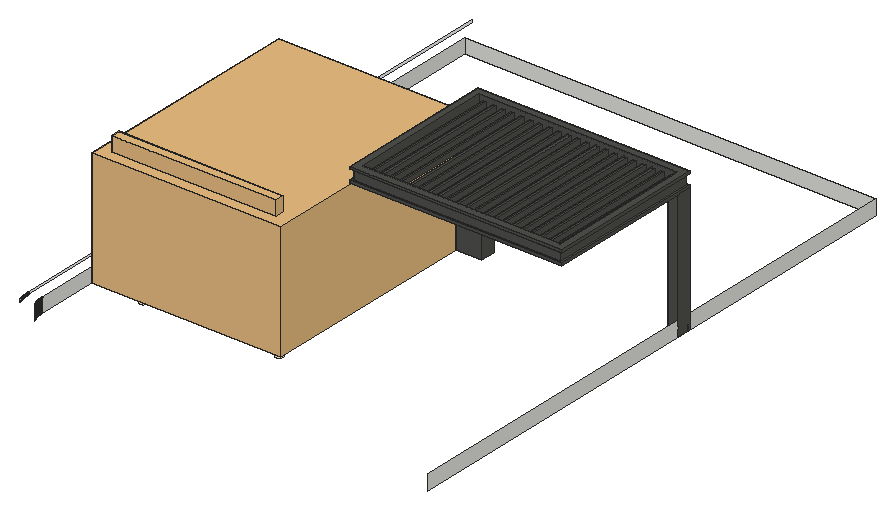
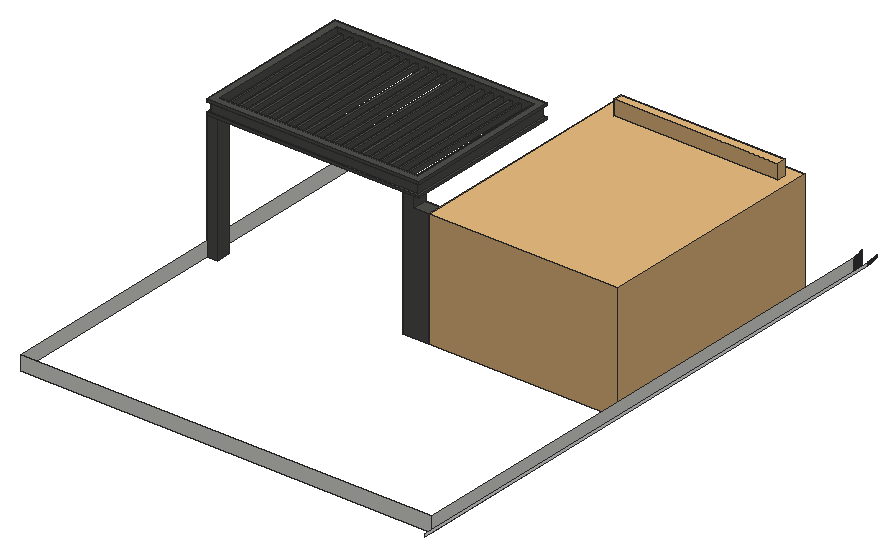
# SketchUp Ruby script. Lengths in inches.
U = 1.inch
M = Sketchup.active_model
def pt(a) = Geom::Point3d.new(a.map { |v| v * U })
def face(e, loops, mat)
  f = e.add_face(loops[0].map { |a| pt(a) })
  loops[1..].each { |l| e.add_face(l.map { |a| pt(a) }).erase! }
  f.material = f.back_material = mat if mat
  f
end
# faces: each face lists its corners as indices into pts; further lists are holes
def faces(e, pts, list, mat = nil) = list.each { |f| face(e, (f[0].is_a?(Array) ? f : [f]).map { |l| l.map { |i| pts[i] } }, mat) }
# xy, xz, yz: faces in a plane at the given z, y or x. An outline is a flat list of corners, or four numbers for a rectangle; further outlines are holes
def ring(l) = l.size == 4 ? [[l[0], l[1]], [l[2], l[1]], [l[2], l[3]], [l[0], l[3]]] : l.each_slice(2).to_a
def flat(e, list, mat, &to3) = list.each { |f| face(e, (f[0].is_a?(Array) ? f : [f]).map { |l| ring(l).map { |u, v| to3.(u, v) } }, mat) }
def xy(e, z, list, mat = nil) = flat(e, list, mat) { |x, y| [x, y, z] }
def xz(e, y, list, mat = nil) = flat(e, list, mat) { |x, z| [x, y, z] }
def yz(e, x, list, mat = nil) = flat(e, list, mat) { |y, z| [x, y, z] }
def lines(e, pts, list) = list.each { |a, b| e.add_line(pt(pts[a]), pt(pts[b])) }
# prism: a flat outline (further loops are holes) pulled along v
def prism(e, loops, v, mat = nil)
  f = face(e, loops, mat); d = Geom::Vector3d.new(v.map { |x| x * U })
  f.pushpull(f.normal.samedirection?(d) ? d.length : -d.length)
end
def box(e, o, s, mat = nil) = prism(e, [[o, [o[0] + s[0], o[1], o[2]], [o[0] + s[0], o[1] + s[1], o[2]], [o[0], o[1] + s[1], o[2]]]], [0, 0, s[2]], mat)
def at(x, y, z, deg = 0) = Geom::Transformation.translation(pt([x, y, z])) * Geom::Transformation.rotation(ORIGIN, Z_AXIS, deg.degrees)
def axes(o, x, y, z) = Geom::Transformation.new([*x, 0, *y, 0, *z, 0, *pt(o).to_a, 1])
def part(name) = M.definitions.add(name)
# library, detail: a bought-in or finely detailed component or shape, given as its bounding box
def library(name, o, s) = part(name).tap { |d| box(d.entities, o, s) }
def detail(e, o, s) = box(e.add_group.entities, o, s)
def put(e, d, t, mat = nil) = e.add_instance(d, t).tap { |i| i.material = mat if mat }
def group(e, t, mat = nil) = e.add_group.tap { |g| g.transformation = t; g.material = mat if mat }.entities
root = M.entities
M.materials.add("1122 AP 7994 PEACH ROSE").color = [254, 227, 201]
M.materials.add("1512 AP 8301 COAL MINE").color = [80, 80, 77]
M.materials.add("[Quartz Light Grey]").color = [251, 251, 252]
c1 = library("Component_63",[0,-41.05,1.35],[7.23,156.73,136.43])
c2 = library("Group\#16",[0,-0.25,0],[156,192.25,96])
c3 = part("3")
box(c3.entities,[1,-120.3125,0],[2.5,120.3125,4])
xy(root,281.82,[[52.82,246,52.75,246.01,52.43,246.05,52.36,246.07,52.28,246.08,52.2,246.1,52.13,246.125,52.05,246.15,51.98,246.17,51.91,246.2,51.83,246.23,51.76,246.26,51.6875,246.29,51.62,246.33,51.55,246.36,51.41,246.44,51.35,246.48,51.28,246.53,51.22,246.57,51.15,246.62,50.97,246.77,50.86,246.88,50.8,246.93,50.6,247.17,50.55,247.24,50.51,247.3,50.46,247.37,50.42,247.43,50.34,247.57,50.31,247.64,50.27,247.71,50.18,247.92,50.15,248,50.13,248.07,50.1,248.15,50.08,248.22,50.0625,248.3,50.05,248.375,50.03,248.45,50.01,248.61,50,248.6875,49.99,248.76,49.99,248.84,49.98,248.92,49.98,249.08,49.99,249.16,49.99,249.24,50,249.3125,50.01,249.39,50.03,249.55,50.05,249.625,50.0625,249.7,50.08,249.78,50.1,249.85,50.13,249.93,50.15,250,50.18,250.08,50.27,250.29,50.31,250.36,50.34,250.43,50.42,250.57,50.46,250.63,50.51,250.7,50.55,250.76,50.6,250.83,50.8,251.07,50.86,251.12,50.97,251.23,51.15,251.38,51.22,251.43,51.28,251.47,51.35,251.52,51.41,251.56,51.55,251.64,51.62,251.67,51.6875,251.71,51.76,251.74,51.83,251.77,51.91,251.8,51.98,251.83,52.05,251.85,52.13,251.875,52.2,251.9,52.28,251.92,52.36,251.93,52.43,251.95,52.75,251.99,52.82,252,53.14,252,53.22,251.99,53.29,251.98,53.53,251.95,53.6,251.93,53.68,251.92,53.76,251.9,53.83,251.875,53.91,251.85,53.98,251.83,54.06,251.8,54.27,251.71,54.34,251.67,54.41,251.64,54.55,251.56,54.61,251.52,54.68,251.47,54.74,251.43,54.81,251.38,55.05,251.18,55.1,251.12,55.16,251.07,55.26,250.95,55.3125,250.89,55.36,250.83,55.41,250.76,55.45,250.7,55.5,250.63,55.54,250.57,55.62,250.43,55.65,250.36,55.6875,250.29,55.72,250.22,55.78,250.08,55.81,250,55.83,249.93,55.86,249.85,55.88,249.78,55.9,249.7,55.92,249.625,55.93,249.55,55.94,249.47,55.96,249.39,55.96,249.3125,55.97,249.24,55.98,249.16,55.98,248.84,55.97,248.76,55.96,248.6875,55.96,248.61,55.94,248.53,55.93,248.45,55.92,248.375,55.9,248.3,55.88,248.22,55.86,248.15,55.83,248.07,55.81,248,55.78,247.92,55.72,247.78,55.6875,247.71,55.65,247.64,55.62,247.57,55.54,247.43,55.5,247.37,55.45,247.3,55.41,247.24,55.36,247.17,55.3125,247.11,55.26,247.05,55.16,246.93,55.1,246.88,55.05,246.82,54.81,246.62,54.74,246.57,54.68,246.53,54.61,246.48,54.55,246.44,54.41,246.36,54.34,246.33,54.27,246.29,54.06,246.2,53.98,246.17,53.91,246.15,53.83,246.125,53.76,246.1,53.68,246.08,53.6,246.07,53.53,246.05,53.29,246.02,53.22,246.01,53.14,246],[164.84,246,164.76,246.01,164.6875,246.02,164.61,246.03,164.45,246.05,164.375,246.07,164.3,246.08,164.22,246.1,164.15,246.125,164.07,246.15,164,246.17,163.92,246.2,163.71,246.29,163.64,246.33,163.57,246.36,163.43,246.44,163.37,246.48,163.3,246.53,163.24,246.57,163.17,246.62,162.93,246.82,162.88,246.88,162.82,246.93,162.62,247.17,162.57,247.24,162.53,247.3,162.48,247.37,162.44,247.43,162.36,247.57,162.33,247.64,162.29,247.71,162.2,247.92,162.17,248,162.15,248.07,162.125,248.15,162.1,248.22,162.08,248.3,162.07,248.375,162.05,248.45,162.03,248.61,162.02,248.6875,162.01,248.76,162,248.84,162,249.16,162.01,249.24,162.02,249.3125,162.03,249.39,162.05,249.55,162.07,249.625,162.08,249.7,162.1,249.78,162.125,249.85,162.15,249.93,162.17,250,162.2,250.08,162.29,250.29,162.33,250.36,162.36,250.43,162.44,250.57,162.48,250.63,162.53,250.7,162.57,250.76,162.62,250.83,162.82,251.07,162.88,251.12,162.93,251.18,163.17,251.38,163.24,251.43,163.3,251.47,163.37,251.52,163.43,251.56,163.57,251.64,163.64,251.67,163.71,251.71,163.92,251.8,164,251.83,164.07,251.85,164.15,251.875,164.22,251.9,164.3,251.92,164.375,251.93,164.45,251.95,164.61,251.97,164.6875,251.98,164.76,251.99,164.84,252,165.16,252,165.24,251.99,165.3125,251.98,165.39,251.97,165.55,251.95,165.625,251.93,165.7,251.92,165.78,251.9,165.85,251.875,165.93,251.85,166,251.83,166.08,251.8,166.29,251.71,166.36,251.67,166.43,251.64,166.57,251.56,166.63,251.52,166.7,251.47,166.76,251.43,166.83,251.38,167.07,251.18,167.12,251.12,167.18,251.07,167.38,250.83,167.43,250.76,167.47,250.7,167.52,250.63,167.56,250.57,167.64,250.43,167.67,250.36,167.71,250.29,167.8,250.08,167.83,250,167.85,249.93,167.875,249.85,167.9,249.78,167.92,249.7,167.93,249.625,167.95,249.55,167.97,249.39,167.98,249.3125,167.99,249.24,168,249.16,168,248.84,167.99,248.76,167.98,248.6875,167.97,248.61,167.95,248.45,167.93,248.375,167.92,248.3,167.9,248.22,167.875,248.15,167.85,248.07,167.83,248,167.8,247.92,167.71,247.71,167.67,247.64,167.64,247.57,167.56,247.43,167.52,247.37,167.47,247.3,167.43,247.24,167.38,247.17,167.18,246.93,167.12,246.88,167.07,246.82,166.83,246.62,166.76,246.57,166.7,246.53,166.63,246.48,166.57,246.44,166.43,246.36,166.36,246.33,166.29,246.29,166.08,246.2,166,246.17,165.93,246.15,165.85,246.125,165.78,246.1,165.7,246.08,165.625,246.07,165.55,246.05,165.39,246.03,165.3125,246.02,165.24,246.01,165.16,246]],"1122 AP 7994 PEACH ROSE")
xz(root,624,[[18,287.82,357,299.82]])
yz(root,7,[[188.67,297.82,189,299.82],[189,297.82,645,299.82]],"[Quartz Light Grey]")
yz(root,7.01,[[188.01,297.82,188.34,299.82]],"[Quartz Light Grey]")
yz(root,18,[[188.53,287.82,188.76,299.82],[188.76,287.82,189,299.82],[189,287.82,624,299.82]])
yz(root,357,[[162,287.82,624,299.82]])
p = [[20.63,177.375,287.82],[20.53,177.59,287.82],[20.53,177.59,299.82],[20.63,177.375,299.82],[20.43,177.8,287.82],[20.43,177.8,299.82],
  [20.33,178.02,287.82],[20.33,178.02,299.82],[20.24,178.23,287.82],[20.24,178.23,299.82],[20.15,178.45,287.82],[20.15,178.45,299.82],
  [20.06,178.67,287.82],[20.06,178.67,299.82],[19.97,178.89,287.82],[19.97,178.89,299.82],[19.88,179.1,287.82],[19.88,179.1,299.82],
  [19.79,179.32,287.82],[19.79,179.32,299.82],[19.71,179.54,287.82],[19.71,179.54,299.82],[19.63,179.77,287.82],[19.63,179.77,299.82],
  [19.55,179.99,287.82],[19.55,179.99,299.82],[19.47,180.21,287.82],[19.47,180.21,299.82],[19.4,180.43,287.82],[19.4,180.43,299.82],
  [19.32,180.66,287.82],[19.32,180.66,299.82],[19.25,180.88,287.82],[19.25,180.88,299.82],[19.18,181.11,287.82],[19.18,181.11,299.82],
  [19.11,181.33,287.82],[19.11,181.33,299.82],[19.05,181.56,287.82],[19.05,181.56,299.82],[18.98,181.78,287.82],[18.98,181.78,299.82],
  [18.92,182.01,287.82],[18.92,182.01,299.82],[18.86,182.24,287.82],[18.86,182.24,299.82],[18.8,182.47,287.82],[18.8,182.47,299.82],
  [18.75,182.7,287.82],[18.75,182.7,299.82],[18.69,182.93,287.82],[18.69,182.93,299.82],[18.64,183.16,287.82],[18.64,183.16,299.82],
  [18.59,183.39,287.82],[18.59,183.39,299.82],[18.54,183.62,287.82],[18.54,183.62,299.82],[18.5,183.85,287.82],[18.5,183.85,299.82],
  [18.45,184.08,287.82],[18.45,184.08,299.82],[18.41,184.3125,287.82],[18.41,184.3125,299.82],[18.37,184.54,287.82],[18.37,184.54,299.82],
  [18.33,184.78,287.82],[18.33,184.78,299.82],[18.3,185.01,287.82],[18.3,185.01,299.82],[18.26,185.24,287.82],[18.26,185.24,299.82],
  [18.23,185.48,287.82],[18.23,185.48,299.82],[18.2,185.71,287.82],[18.2,185.71,299.82],[18.17,185.94,287.82],[18.17,185.94,299.82],
  [18.15,186.18,287.82],[18.15,186.18,299.82],[18.125,186.41,287.82],[18.125,186.41,299.82],[18.1,186.65,287.82],[18.1,186.65,299.82],
  [18.08,186.88,287.82],[18.08,186.88,299.82],[18.07,187.12,287.82],[18.07,187.12,299.82],[18.05,187.35,287.82],[18.05,187.35,299.82],
  [18.04,187.59,287.82],[18.04,187.59,299.82],[18.03,187.82,287.82],[18.03,187.82,299.82],[18.02,188.06,287.82],[18.02,188.06,299.82],
  [18.01,188.29,287.82],[18.01,188.29,299.82],[18,188.53,287.82],[18,188.53,299.82],[8.66,177.89,299.82],[8.66,177.89,297.82],
  [8.76,177.57,297.82],[8.76,177.57,299.82],[8.56,178.21,299.82],[8.56,178.21,297.82],[8.47,178.53,299.82],[8.47,178.53,297.82],
  [8.38,178.84,299.82],[8.38,178.84,297.82],[8.29,179.16,299.82],[8.29,179.16,297.82],[8.21,179.49,299.82],[8.21,179.49,297.82],
  [8.13,179.81,299.82],[8.13,179.81,297.82],[8.05,180.13,299.82],[8.05,180.13,297.82],[7.97,180.45,299.82],[7.97,180.45,297.82],
  [7.9,180.78,299.82],[7.9,180.78,297.82],[7.83,181.1,299.82],[7.83,181.1,297.82],[7.76,181.42,299.82],[7.76,181.42,297.82],
  [7.7,181.75,299.82],[7.7,181.75,297.82],[7.64,182.08,299.82],[7.64,182.08,297.82],[7.58,182.4,299.82],[7.58,182.4,297.82],
  [7.52,182.73,299.82],[7.52,182.73,297.82],[7.47,183.06,299.82],[7.47,183.06,297.82],[7.42,183.38,299.82],[7.42,183.38,297.82],
  [7.37,183.71,299.82],[7.37,183.71,297.82],[7.33,184.04,299.82],[7.33,184.04,297.82],[7.28,184.37,299.82],[7.28,184.37,297.82],
  [7.24,184.7,299.82],[7.24,184.7,297.82],[7.21,185.03,299.82],[7.21,185.03,297.82],[7.17,185.36,299.82],[7.17,185.36,297.82],
  [7.14,185.6875,299.82],[7.14,185.6875,297.82],[7.12,186.02,299.82],[7.12,186.02,297.82],[7.09,186.35,299.82],[7.09,186.35,297.82],
  [7.07,186.68,299.82],[7.07,186.68,297.82],[7.05,187.01,299.82],[7.05,187.01,297.82],[7.04,187.34,299.82],[7.04,187.34,297.82],
  [7.02,187.67,299.82],[7.02,187.67,297.82],[7.01,188.01,299.82],[7.01,188.01,297.82],[7,188.67,299.82],[7,188.67,297.82],
  [7.01,188.34,297.82],[7.01,188.34,299.82]]
faces(root,p,[[0,1,2,3],[1,4,5,2],[4,6,7,5],[6,8,9,7],[8,10,11,9],[10,12,13,11],[12,14,15,13],[14,16,17,15],
  [16,18,19,17],[18,20,21,19],[20,22,23,21],[22,24,25,23],[24,26,27,25],[26,28,29,27],[28,30,31,29],[30,32,33,31],
  [32,34,35,33],[34,36,37,35],[36,38,39,37],[38,40,41,39],[40,42,43,41],[42,44,45,43],[44,46,47,45],[46,48,49,47],
  [48,50,51,49],[50,52,53,51],[52,54,55,53],[54,56,57,55],[56,58,59,57],[58,60,61,59],[60,62,63,61],[62,64,65,63],
  [64,66,67,65],[66,68,69,67],[68,70,71,69],[70,72,73,71],[72,74,75,73],[74,76,77,75],[76,78,79,77],[78,80,81,79],
  [80,82,83,81],[82,84,85,83],[84,86,87,85],[86,88,89,87],[88,90,91,89],[90,92,93,91],[92,94,95,93],[94,96,97,95],
  [96,98,99,97]])
faces(root,p,[[100,101,102,103],[104,105,101,100],[106,107,105,104],[108,109,107,106],[110,111,109,108],[112,113,111,110],[114,115,113,112],[116,117,115,114],
  [118,119,117,116],[120,121,119,118],[122,123,121,120],[124,125,123,122],[126,127,125,124],[128,129,127,126],[130,131,129,128],[132,133,131,130],
  [134,135,133,132],[136,137,135,134],[138,139,137,136],[140,141,139,138],[142,143,141,140],[144,145,143,142],[146,147,145,144],[148,149,147,146],
  [150,151,149,148],[152,153,151,150],[154,155,153,152],[156,157,155,154],[158,159,157,156],[160,161,159,158],[162,163,161,160],[164,165,163,162],
  [166,167,168,169]],"[Quartz Light Grey]")
put(root,c1,axes([126.64,249,396.67],[0,1,0],[-0.86133,0,0],[0,0,-0.79]))
put(root,c2,at(18,240,287.82))
g1 = group(root,at(174,420,287.82),"1512 AP 8301 COAL MINE")
xy(g1,105,[[[7.99,-120,183,12.3125],[13.99,-114,177,6.3125]]])
xy(g1,107,[[[7.99,-120,183,12.3125],[9.99,-118,181,10.3125]]])
xy(g1,115,[[[7.99,-120,183,12.3125],[9.99,-118,181,10.3125]]])
xy(g1,117,[[[7.99,-120,183,12.3125],[13.99,-114,177,6.3125]]])
xz(g1,-120,[[7.99,105,183,107],[7.99,115,183,117]])
xz(g1,-118,[[9.99,107,181,115]])
xz(g1,-114,[[13.99,105,177,117]])
xz(g1,6.3125,[[13.99,105,177,117]])
xz(g1,10.3125,[[9.99,107,181,115]])
xz(g1,12.3125,[[7.99,105,183,107],[7.99,115,183,117]])
yz(g1,7.99,[[-120,105,12.3125,107],[-120,115,12.3125,117]])
yz(g1,9.99,[[-118,107,10.3125,115]])
yz(g1,13.99,[[-114,105,6.3125,117]])
yz(g1,177,[[-114,105,6.3125,117]])
yz(g1,181,[[-118,107,10.3125,115]])
yz(g1,183,[[-120,105,12.3125,107],[-120,115,12.3125,117]])
put(g1,c3,at(170.5,6.3125,109))
put(g1,c3,at(162.77,6.3125,109))
put(g1,c3,at(155.05,6.3125,109))
put(g1,c3,at(147.32,6.3125,109))
put(g1,c3,at(139.6,6.3125,109))
put(g1,c3,at(131.875,6.3125,109))
put(g1,c3,at(124.15,6.3125,109))
put(g1,c3,at(116.42,6.3125,109))
put(g1,c3,at(108.7,6.3125,109))
put(g1,c3,at(100.97,6.3125,109))
put(g1,c3,at(93.25,6.3125,109))
put(g1,c3,at(85.52,6.3125,109))
put(g1,c3,at(77.8,6.3125,109))
put(g1,c3,at(70.07,6.3125,109))
put(g1,c3,at(62.35,6.3125,109))
put(g1,c3,at(54.62,6.3125,109))
put(g1,c3,at(46.9,6.3125,109))
put(g1,c3,at(39.17,6.3125,109))
put(g1,c3,at(31.44,6.3125,109))
put(g1,c3,at(23.72,6.3125,109))
put(g1,c3,at(15.99,6.3125,109))
g2 = group(g1,at(162,0,0))
xy(g2,0,[[12,0,21,12]])
xy(g2,105,[[12,0,21,12]])
xz(g2,0,[[12,0,21,105]])
xz(g2,12,[[12,0,21,105]])
yz(g2,12,[[0,0,12,105]])
yz(g2,21,[[0,0,12,105]])
p = [[12,12,96],[12,12.47,96]]
lines(g2,p,[[0,1]])
g3 = group(g1,at(0,0,0))
prism(g3,[[[21,12,0],[0,12,0],[0,12,96],[12,12,96],[12,12,105],[21,12,105]]],[0,-12,0])
p = [[12,12,96],[12,12.47,96]]
lines(g3,p,[[0,1]])
